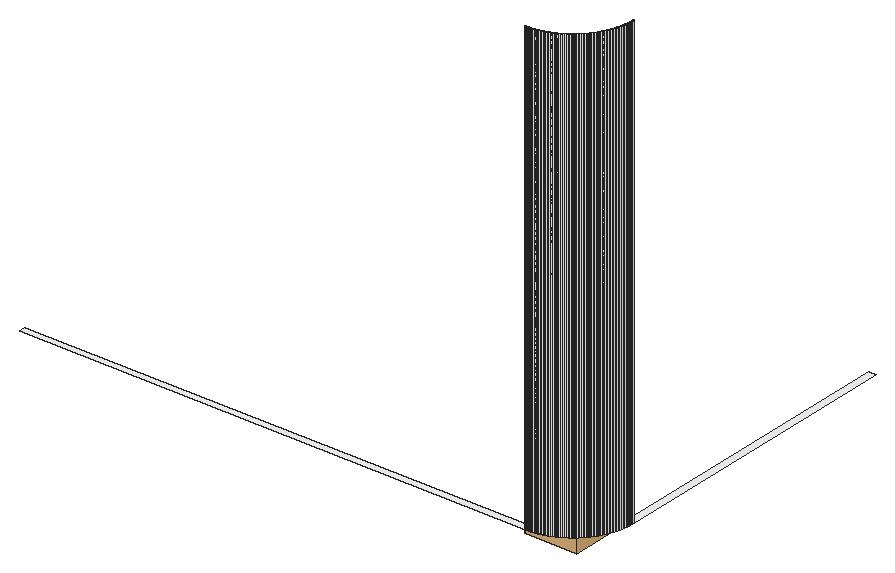
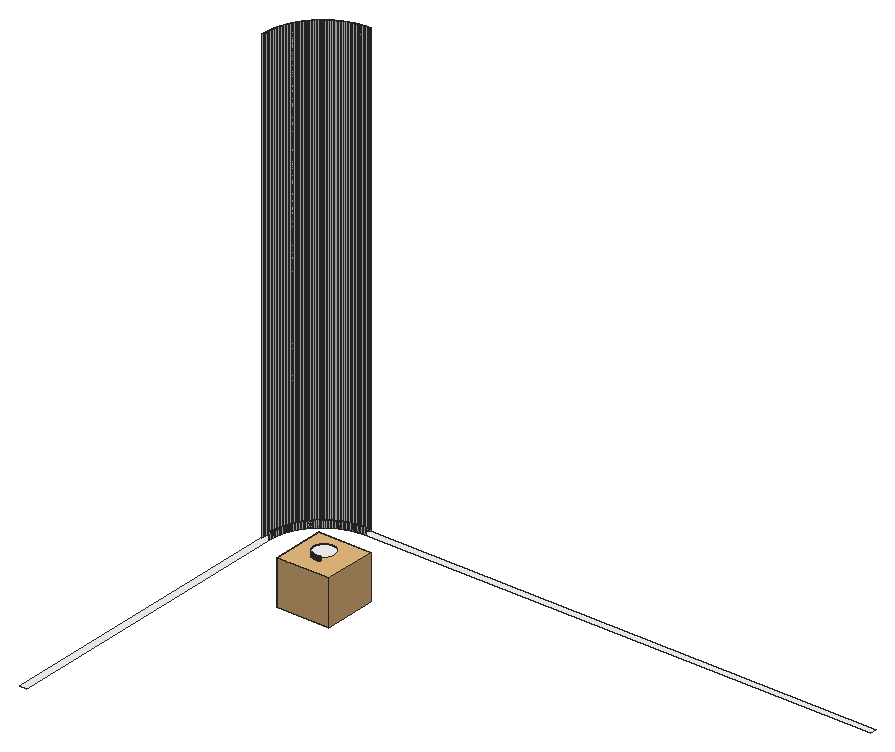
# SketchUp Ruby script. Lengths in inches.
U = 1.inch
M = Sketchup.active_model
def pt(a) = Geom::Point3d.new(a.map { |v| v * U })
def face(e, loops, mat)
  f = e.add_face(loops[0].map { |a| pt(a) })
  loops[1..].each { |l| e.add_face(l.map { |a| pt(a) }).erase! }
  f.material = f.back_material = mat if mat
  f
end
# faces: each face lists its corners as indices into pts; further lists are holes
def faces(e, pts, list, mat = nil) = list.each { |f| face(e, (f[0].is_a?(Array) ? f : [f]).map { |l| l.map { |i| pts[i] } }, mat) }
# xy, xz, yz: faces in a plane at the given z, y or x. An outline is a flat list of corners, or four numbers for a rectangle; further outlines are holes
def ring(l) = l.size == 4 ? [[l[0], l[1]], [l[2], l[1]], [l[2], l[3]], [l[0], l[3]]] : l.each_slice(2).to_a
def flat(e, list, mat, &to3) = list.each { |f| face(e, (f[0].is_a?(Array) ? f : [f]).map { |l| ring(l).map { |u, v| to3.(u, v) } }, mat) }
def xy(e, z, list, mat = nil) = flat(e, list, mat) { |x, y| [x, y, z] }
def xz(e, y, list, mat = nil) = flat(e, list, mat) { |x, z| [x, y, z] }
def yz(e, x, list, mat = nil) = flat(e, list, mat) { |y, z| [x, y, z] }
def lines(e, pts, list) = list.each { |a, b| e.add_line(pt(pts[a]), pt(pts[b])) }
# prism: a flat outline (further loops are holes) pulled along v
def prism(e, loops, v, mat = nil)
  f = face(e, loops, mat); d = Geom::Vector3d.new(v.map { |x| x * U })
  f.pushpull(f.normal.samedirection?(d) ? d.length : -d.length)
end
def box(e, o, s, mat = nil) = prism(e, [[o, [o[0] + s[0], o[1], o[2]], [o[0] + s[0], o[1] + s[1], o[2]], [o[0], o[1] + s[1], o[2]]]], [0, 0, s[2]], mat)
def at(x, y, z, deg = 0) = Geom::Transformation.translation(pt([x, y, z])) * Geom::Transformation.rotation(ORIGIN, Z_AXIS, deg.degrees)
def axes(o, x, y, z) = Geom::Transformation.new([*x, 0, *y, 0, *z, 0, *pt(o).to_a, 1])
def part(name) = M.definitions.add(name)
# library, detail: a bought-in or finely detailed component or shape, given as its bounding box
def library(name, o, s) = part(name).tap { |d| box(d.entities, o, s) }
def detail(e, o, s) = box(e.add_group.entities, o, s)
def put(e, d, t, mat = nil) = e.add_instance(d, t).tap { |i| i.material = mat if mat }
def group(e, t, mat = nil) = e.add_group.tap { |g| g.transformation = t; g.material = mat if mat }.entities
root = M.entities
M.materials.add("[Quartz Light Grey]").color = [251, 251, 252]
c1 = library("5",[-6.25,-6.25,-13.16],[15.58,15.58,13.16])
xy(root,115,[[60,187,60,189,210.21,189,210.42,189.01,210.63,189.01,211.05,189.03,211.26,189.05,211.46,189.07,211.88,189.11,212.3,189.17,212.5,189.2,212.71,189.23,212.92,189.27,213.12,189.31,213.33,189.35,213.53,189.39,213.74,189.44,213.9375,189.49,214.14,189.55,214.34,189.6,214.94,189.78,215.54,189.99,215.73,190.0625,215.93,190.14,216.12,190.22,216.32,190.3,216.51,190.38,217.08,190.65,217.26,190.74,217.45,190.84,217.63,190.9375,217.82,191.04,218,191.14,218.54,191.47,218.71,191.58,218.89,191.7,219.0625,191.8125,219.23,191.93,219.4,192.06,219.57,192.18,219.74,192.31,219.91,192.43,220.07,192.57,220.39,192.83,220.71,193.11,221.01,193.39,221.16,193.54,221.3125,193.6875,221.46,193.84,221.61,193.99,221.89,194.29,222.17,194.61,222.43,194.93,222.57,195.09,222.69,195.26,222.82,195.43,222.94,195.6,223.07,195.77,223.1875,195.9375,223.3,196.11,223.42,196.29,223.53,196.46,223.86,197,223.96,197.18,224.0625,197.37,224.16,197.55,224.26,197.74,224.35,197.92,224.62,198.49,224.7,198.68,224.78,198.88,224.86,199.07,224.9375,199.27,225.01,199.46,225.22,200.06,225.4,200.66,225.45,200.86,225.51,201.0625,225.56,201.26,225.61,201.47,225.65,201.67,225.69,201.88,225.73,202.08,225.77,202.29,225.8,202.5,225.83,202.7,225.89,203.12,225.93,203.54,225.95,203.74,225.97,203.95,225.99,204.37,225.99,204.58,226,204.79,226,295,228,295,228,204.76,227.99,204.53,227.99,204.29,227.98,204.06,227.96,203.82,227.94,203.59,227.92,203.35,227.9,203.12,227.875,202.88,227.85,202.65,227.8125,202.42,227.78,202.18,227.7,201.72,227.65,201.49,227.61,201.26,227.56,201.03,227.5,200.8,227.45,200.57,227.39,200.34,227.32,200.11,227.26,199.89,227.19,199.66,227.12,199.4375,227.04,199.21,226.97,198.99,226.89,198.77,226.8,198.55,226.72,198.33,226.54,197.89,226.44,197.68,226.35,197.46,226.25,197.25,226.14,197.04,226.04,196.83,225.82,196.41,225.7,196.2,225.59,196,225.35,195.6,225.22,195.39,225.1,195.2,224.97,195,224.83,194.8,224.7,194.61,224.5625,194.42,224.42,194.23,224.28,194.04,224.14,193.86,223.99,193.67,223.84,193.49,223.6875,193.31,223.53,193.13,223.375,192.96,223.22,192.78,223.06,192.61,222.89,192.44,222.73,192.27,222.56,192.11,222.39,191.94,222.22,191.78,222.04,191.625,221.87,191.47,221.69,191.3125,221.51,191.16,221.33,191.01,221.14,190.86,220.96,190.72,220.77,190.58,220.58,190.4375,220.39,190.3,220.2,190.17,220,190.03,219.8,189.9,219.61,189.78,219.4,189.65,219,189.41,218.8,189.3,218.59,189.18,218.17,188.96,217.96,188.86,217.75,188.75,217.54,188.65,217.32,188.56,217.11,188.46,216.67,188.28,216.45,188.2,216.23,188.11,216.01,188.03,215.79,187.96,215.5625,187.88,215.34,187.81,215.11,187.74,214.89,187.68,214.66,187.61,214.43,187.55,214.2,187.5,213.97,187.44,213.74,187.39,213.51,187.35,213.28,187.3,212.82,187.22,212.58,187.1875,212.35,187.15,212.12,187.125,211.88,187.1,211.65,187.08,211.41,187.06,211.18,187.04,210.94,187.02,210.71,187.01,210.47,187.01,210.24,187]],"[Quartz Light Grey]")
xy(root,119.5,[[207.84,204,207.76,204.01,207.6875,204.02,207.61,204.03,207.45,204.05,207.375,204.07,207.3,204.08,207.22,204.1,207.15,204.125,207.07,204.15,207,204.17,206.92,204.2,206.71,204.29,206.64,204.33,206.57,204.36,206.43,204.44,206.37,204.48,206.3,204.53,206.24,204.57,206.17,204.62,205.93,204.82,205.88,204.88,205.82,204.93,205.62,205.17,205.57,205.24,205.53,205.3,205.48,205.37,205.44,205.43,205.36,205.57,205.33,205.64,205.29,205.71,205.2,205.92,205.17,206,205.15,206.07,205.125,206.15,205.1,206.22,205.08,206.3,205.07,206.375,205.05,206.45,205.03,206.61,205.02,206.6875,205.01,206.76,205,206.84,205,207.16,205.01,207.24,205.02,207.3125,205.03,207.39,205.05,207.55,205.07,207.625,205.08,207.7,205.1,207.78,205.125,207.85,205.15,207.93,205.17,208,205.2,208.08,205.29,208.29,205.33,208.36,205.36,208.43,205.44,208.57,205.48,208.63,205.53,208.7,205.57,208.76,205.62,208.83,205.82,209.07,205.88,209.12,205.93,209.18,206.17,209.38,206.24,209.43,206.3,209.47,206.37,209.52,206.43,209.56,206.57,209.64,206.64,209.67,206.71,209.71,206.92,209.8,207,209.83,207.07,209.85,207.15,209.875,207.22,209.9,207.3,209.92,207.375,209.93,207.45,209.95,207.61,209.97,207.6875,209.98,207.76,209.99,207.84,210,208.16,210,208.24,209.99,208.3125,209.98,208.39,209.97,208.55,209.95,208.625,209.93,208.7,209.92,208.78,209.9,208.85,209.875,208.93,209.85,209,209.83,209.08,209.8,209.29,209.71,209.36,209.67,209.43,209.64,209.57,209.56,209.63,209.52,209.7,209.47,209.76,209.43,209.83,209.38,210.07,209.18,210.12,209.12,210.18,209.07,210.38,208.83,210.43,208.76,210.47,208.7,210.52,208.63,210.56,208.57,210.64,208.43,210.67,208.36,210.71,208.29,210.8,208.08,210.83,208,210.85,207.93,210.875,207.85,210.9,207.78,210.92,207.7,210.93,207.625,210.95,207.55,210.97,207.39,210.98,207.3125,210.99,207.24,211,207.16,211,206.84,210.99,206.76,210.98,206.6875,210.97,206.61,210.95,206.45,210.93,206.375,210.92,206.3,210.9,206.22,210.875,206.15,210.85,206.07,210.83,206,210.8,205.92,210.71,205.71,210.67,205.64,210.64,205.57,210.56,205.43,210.52,205.37,210.47,205.3,210.43,205.24,210.38,205.17,210.18,204.93,210.12,204.88,210.07,204.82,209.83,204.62,209.76,204.57,209.7,204.53,209.63,204.48,209.57,204.44,209.43,204.36,209.36,204.33,209.29,204.29,209.08,204.2,209,204.17,208.93,204.15,208.85,204.125,208.78,204.1,208.7,204.08,208.625,204.07,208.55,204.05,208.39,204.03,208.3125,204.02,208.24,204.01,208.16,204]],"[Quartz Light Grey]")
xz(root,187,[[210,115,210.24,249]],"[Quartz Light Grey]")
xz(root,187.01,[[210.47,115,210.71,249]],"[Quartz Light Grey]")
xz(root,189,[[210,115,210.21,117]],"[Quartz Light Grey]")
xz(root,189.01,[[210.42,115,210.63,117]],"[Quartz Light Grey]")
xz(root,204,[[207.84,117,207.92,119.5],[207.92,117,208,119.5],[208,117,208.08,119.5],[208.08,117,208.16,119.5]],"[Quartz Light Grey]")
xz(root,210,[[207.84,117,207.92,119.5],[207.92,117,208,119.5],[208,117,208.08,119.5],[208.08,117,208.16,119.5]],"[Quartz Light Grey]")
yz(root,211,[[206.84,117,206.92,119.5],[206.92,117,207,119.5],[207,117,207.08,119.5],[207.08,117,207.16,119.5]],"[Quartz Light Grey]")
yz(root,225.99,[[204.37,115,204.58,117]],"[Quartz Light Grey]")
yz(root,226,[[204.79,115,205,117]],"[Quartz Light Grey]")
yz(root,227.99,[[204.29,115,204.53,249]],"[Quartz Light Grey]")
yz(root,228,[[204.76,115,205,249]],"[Quartz Light Grey]")
p = [[210.24,187,115],[210.47,187.01,115],[210.47,187.01,249],[210.24,187,249],[210.71,187.01,115],[210.94,187.02,115],
  [210.94,187.02,249],[210.71,187.01,249],[211.18,187.04,115],[211.18,187.04,249],[211.41,187.06,115],[211.41,187.06,249],
  [211.65,187.08,115],[211.65,187.08,249],[211.88,187.1,115],[211.88,187.1,249],[212.12,187.125,115],[212.12,187.125,249],
  [212.35,187.15,115],[212.35,187.15,249],[212.58,187.1875,115],[212.58,187.1875,249],[212.82,187.22,115],[212.82,187.22,249],
  [213.05,187.26,115],[213.05,187.26,249],[213.28,187.3,115],[213.28,187.3,249],[213.51,187.35,115],[213.51,187.35,249],
  [213.74,187.39,115],[213.74,187.39,249],[213.97,187.44,115],[213.97,187.44,249],[214.2,187.5,115],[214.2,187.5,249],
  [214.43,187.55,115],[214.43,187.55,249],[214.66,187.61,115],[214.66,187.61,249],[214.89,187.68,115],[214.89,187.68,249],
  [215.11,187.74,115],[215.11,187.74,249],[215.34,187.81,115],[215.34,187.81,249],[215.5625,187.88,115],[215.5625,187.88,249],
  [215.79,187.96,115],[215.79,187.96,249],[216.01,188.03,115],[216.01,188.03,249],[216.23,188.11,115],[216.23,188.11,249],
  [216.45,188.2,115],[216.45,188.2,249],[216.67,188.28,115],[216.67,188.28,249],[216.89,188.37,115],[216.89,188.37,249],
  [217.11,188.46,115],[217.11,188.46,249],[217.32,188.56,115],[217.32,188.56,249],[217.54,188.65,115],[217.54,188.65,249],
  [217.75,188.75,115],[217.75,188.75,249],[217.96,188.86,115],[217.96,188.86,249],[218.17,188.96,115],[218.17,188.96,249],
  [210.42,189.01,115],[210.21,189,115],[210.21,189,117],[210.42,189.01,117],[210.84,189.02,115],[210.63,189.01,115],
  [210.63,189.01,117],[210.84,189.02,117],[211.05,189.03,115],[211.05,189.03,117],[211.26,189.05,115],[211.26,189.05,117],
  [211.46,189.07,115],[211.46,189.07,117],[218.38,189.07,115],[218.38,189.07,249],[211.67,189.09,115],[211.67,189.09,117],
  [211.88,189.11,115],[211.88,189.11,117],[212.09,189.14,115],[212.09,189.14,117],[212.3,189.17,115],[212.3,189.17,117],
  [218.59,189.18,115],[218.59,189.18,249],[212.5,189.2,115],[212.5,189.2,117],[212.71,189.23,115],[212.71,189.23,117],
  [212.92,189.27,115],[212.92,189.27,117],[218.8,189.3,115],[218.8,189.3,249],[213.12,189.31,115],[213.12,189.31,117],
  [213.33,189.35,115],[213.33,189.35,117],[213.53,189.39,115],[213.53,189.39,117],[219,189.41,115],[219,189.41,249],
  [213.74,189.44,115],[213.74,189.44,117],[213.9375,189.49,115],[213.9375,189.49,117],[219.2,189.53,115],[219.2,189.53,249],
  [214.14,189.55,115],[214.14,189.55,117],[214.34,189.6,115],[214.34,189.6,117],[219.4,189.65,115],[219.4,189.65,249],
  [214.54,189.66,115],[214.54,189.66,117],[214.74,189.72,115],[214.74,189.72,117],[214.94,189.78,115],[214.94,189.78,117],
  [219.61,189.78,115],[219.61,189.78,249],[215.14,189.85,115],[215.14,189.85,117],[215.34,189.92,115],[215.34,189.92,117],
  [219.8,189.9,115],[219.8,189.9,249],[215.54,189.99,115],[215.54,189.99,117],[220,190.03,115],[220,190.03,249],
  [215.73,190.0625,115],[215.73,190.0625,117],[220.2,190.17,115],[220.2,190.17,249],[215.93,190.14,115],[215.93,190.14,117],
  [216.12,190.22,115],[216.12,190.22,117],[216.32,190.3,115],[216.32,190.3,117],[220.39,190.3,115],[220.39,190.3,249],
  [216.51,190.38,115],[216.51,190.38,117],[220.58,190.4375,115],[220.58,190.4375,249],[216.7,190.47,115],[216.7,190.47,117],
  [220.77,190.58,115],[220.77,190.58,249],[216.89,190.56,115],[216.89,190.56,117],[217.08,190.65,115],[217.08,190.65,117],
  [220.96,190.72,115],[220.96,190.72,249],[217.26,190.74,115],[217.26,190.74,117],[217.45,190.84,115],[217.45,190.84,117],
  [221.14,190.86,115],[221.14,190.86,249],[217.63,190.9375,115],[217.63,190.9375,117],[217.82,191.04,115],[217.82,191.04,117],
  [221.33,191.01,115],[221.33,191.01,249],[218,191.14,115],[218,191.14,117],[221.51,191.16,115],[221.51,191.16,249],
  [218.18,191.25,115],[218.18,191.25,117],[218.36,191.36,115],[218.36,191.36,117],[221.69,191.3125,115],[221.69,191.3125,249],
  [221.87,191.47,115],[221.87,191.47,249],[218.54,191.47,115],[218.54,191.47,117],[218.71,191.58,115],[218.71,191.58,117],
  [222.04,191.625,115],[222.04,191.625,249],[218.89,191.7,115],[218.89,191.7,117],[222.22,191.78,115],[222.22,191.78,249],
  [219.0625,191.8125,115],[219.0625,191.8125,117],[219.23,191.93,115],[219.23,191.93,117],[222.39,191.94,115],[222.39,191.94,249],
  [219.4,192.06,115],[219.4,192.06,117],[222.56,192.11,115],[222.56,192.11,249],[219.57,192.18,115],[219.57,192.18,117],
  [222.73,192.27,115],[222.73,192.27,249],[219.74,192.31,115],[219.74,192.31,117],[219.91,192.43,115],[219.91,192.43,117],
  [222.89,192.44,115],[222.89,192.44,249],[220.07,192.57,115],[220.07,192.57,117],[223.06,192.61,115],[223.06,192.61,249],
  [220.23,192.7,115],[220.23,192.7,117],[223.22,192.78,115],[223.22,192.78,249],[220.39,192.83,115],[220.39,192.83,117],
  [220.55,192.97,115],[220.55,192.97,117],[223.375,192.96,115],[223.375,192.96,249],[220.71,193.11,115],[220.71,193.11,117],
  [223.53,193.13,115],[223.53,193.13,249],[220.86,193.25,115],[220.86,193.25,117],[223.6875,193.31,115],[223.6875,193.31,249],
  [221.01,193.39,115],[221.01,193.39,117],[223.84,193.49,115],[223.84,193.49,249],[221.16,193.54,115],[221.16,193.54,117],
  [221.3125,193.6875,115],[221.3125,193.6875,117],[223.99,193.67,115],[223.99,193.67,249],[221.46,193.84,115],[221.46,193.84,117],
  [224.14,193.86,115],[224.14,193.86,249],[221.61,193.99,115],[221.61,193.99,117],[224.28,194.04,115],[224.28,194.04,249],
  [221.75,194.14,115],[221.75,194.14,117],[224.42,194.23,115],[224.42,194.23,249],[221.89,194.29,115],[221.89,194.29,117],
  [224.5625,194.42,115],[224.5625,194.42,249],[222.03,194.45,115],[222.03,194.45,117],[224.7,194.61,115],[224.7,194.61,249],
  [222.17,194.61,115],[222.17,194.61,117],[222.3,194.77,115],[222.3,194.77,117],[224.83,194.8,115],[224.83,194.8,249],
  [222.43,194.93,115],[222.43,194.93,117],[224.97,195,115],[224.97,195,249],[222.57,195.09,115],[222.57,195.09,117],
  [225.1,195.2,115],[225.1,195.2,249],[222.69,195.26,115],[222.69,195.26,117],[225.22,195.39,115],[225.22,195.39,249],
  [222.82,195.43,115],[222.82,195.43,117],[222.94,195.6,115],[222.94,195.6,117],[225.35,195.6,115],[225.35,195.6,249],
  [223.07,195.77,115],[223.07,195.77,117],[225.47,195.8,115],[225.47,195.8,249],[223.1875,195.9375,115],[223.1875,195.9375,117],
  [225.59,196,115],[225.59,196,249],[223.3,196.11,115],[223.3,196.11,117],[225.7,196.2,115],[225.7,196.2,249],
  [223.42,196.29,115],[223.42,196.29,117],[225.82,196.41,115],[225.82,196.41,249],[223.53,196.46,115],[223.53,196.46,117],
  [225.93,196.62,115],[225.93,196.62,249],[223.64,196.64,115],[223.64,196.64,117],[223.75,196.82,115],[223.75,196.82,117],
  [226.04,196.83,115],[226.04,196.83,249],[223.86,197,115],[223.86,197,117],[226.14,197.04,115],[226.14,197.04,249],
  [223.96,197.18,115],[223.96,197.18,117],[226.25,197.25,115],[226.25,197.25,249],[224.0625,197.37,115],[224.0625,197.37,117],
  [226.35,197.46,115],[226.35,197.46,249],[224.16,197.55,115],[224.16,197.55,117],[226.44,197.68,115],[226.44,197.68,249],
  [224.26,197.74,115],[224.26,197.74,117],[224.35,197.92,115],[224.35,197.92,117],[226.54,197.89,115],[226.54,197.89,249],
  [224.44,198.11,115],[224.44,198.11,117],[226.63,198.11,115],[226.63,198.11,249],[224.53,198.3,115],[224.53,198.3,117],
  [226.72,198.33,115],[226.72,198.33,249],[224.62,198.49,115],[224.62,198.49,117],[226.8,198.55,115],[226.8,198.55,249],
  [224.7,198.68,115],[224.7,198.68,117],[226.89,198.77,115],[226.89,198.77,249],[224.78,198.88,115],[224.78,198.88,117],
  [226.97,198.99,115],[226.97,198.99,249],[224.86,199.07,115],[224.86,199.07,117],[227.04,199.21,115],[227.04,199.21,249],
  [224.9375,199.27,115],[224.9375,199.27,117],[227.12,199.4375,115],[227.12,199.4375,249],[225.01,199.46,115],[225.01,199.46,117],
  [227.19,199.66,115],[227.19,199.66,249],[225.08,199.66,115],[225.08,199.66,117],[225.15,199.86,115],[225.15,199.86,117],
  [227.26,199.89,115],[227.26,199.89,249],[225.22,200.06,115],[225.22,200.06,117],[227.32,200.11,115],[227.32,200.11,249],
  [225.28,200.26,115],[225.28,200.26,117],[227.39,200.34,115],[227.39,200.34,249],[225.34,200.46,115],[225.34,200.46,117],
  [227.45,200.57,115],[227.45,200.57,249],[225.4,200.66,115],[225.4,200.66,117],[227.5,200.8,115],[227.5,200.8,249],
  [225.45,200.86,115],[225.45,200.86,117],[227.56,201.03,115],[227.56,201.03,249],[225.51,201.0625,115],[225.51,201.0625,117],
  [227.61,201.26,115],[227.61,201.26,249],[225.56,201.26,115],[225.56,201.26,117],[225.61,201.47,115],[225.61,201.47,117],
  [227.65,201.49,115],[227.65,201.49,249],[225.65,201.67,115],[225.65,201.67,117],[227.7,201.72,115],[227.7,201.72,249],
  [225.69,201.88,115],[225.69,201.88,117],[227.74,201.95,115],[227.74,201.95,249],[225.73,202.08,115],[225.73,202.08,117],
  [227.78,202.18,115],[227.78,202.18,249],[225.77,202.29,115],[225.77,202.29,117],[227.8125,202.42,115],[227.8125,202.42,249],
  [225.8,202.5,115],[225.8,202.5,117],[227.85,202.65,115],[227.85,202.65,249],[225.83,202.7,115],[225.83,202.7,117],
  [225.86,202.91,115],[225.86,202.91,117],[227.875,202.88,115],[227.875,202.88,249],[225.89,203.12,115],[225.89,203.12,117],
  [227.9,203.12,115],[227.9,203.12,249],[225.91,203.33,115],[225.91,203.33,117],[227.92,203.35,115],[227.92,203.35,249],
  [225.93,203.54,115],[225.93,203.54,117],[227.94,203.59,115],[227.94,203.59,249],[225.95,203.74,115],[225.95,203.74,117],
  [227.96,203.82,115],[227.96,203.82,249],[225.97,203.95,115],[225.97,203.95,117],[227.98,204.06,115],[227.98,204.06,249],
  [225.98,204.16,115],[225.98,204.16,117],[227.99,204.29,115],[227.99,204.29,249],[225.99,204.37,115],[225.99,204.37,117],
  [227.99,204.53,115],[228,204.76,115],[228,204.76,249],[227.99,204.53,249],[226,204.79,115],[225.99,204.58,115],
  [225.99,204.58,117],[226,204.79,117],[207.53,204.04,117],[207.45,204.05,117],[207.45,204.05,119.5],[207.53,204.04,119.5],
  [207.61,204.03,117],[207.61,204.03,119.5],[207.6875,204.02,117],[207.6875,204.02,119.5],[207.76,204.01,117],[207.76,204.01,119.5],
  [207.84,204,117],[207.84,204,119.5],[208.24,204.01,117],[208.16,204,117],[208.16,204,119.5],[208.24,204.01,119.5],
  [208.3125,204.02,117],[208.3125,204.02,119.5],[208.39,204.03,117],[208.39,204.03,119.5],[208.47,204.04,117],[208.47,204.04,119.5],
  [208.55,204.05,117],[208.55,204.05,119.5],[207.07,204.15,117],[207,204.17,117],[207,204.17,119.5],[207.07,204.15,119.5],
  [207.15,204.125,117],[207.15,204.125,119.5],[207.22,204.1,117],[207.22,204.1,119.5],[207.3,204.08,117],[207.3,204.08,119.5],
  [207.375,204.07,117],[207.375,204.07,119.5],[208.625,204.07,117],[208.625,204.07,119.5],[208.7,204.08,117],[208.7,204.08,119.5],
  [208.78,204.1,117],[208.78,204.1,119.5],[208.85,204.125,117],[208.85,204.125,119.5],[208.93,204.15,117],[208.93,204.15,119.5],
  [209,204.17,117],[209,204.17,119.5],[206.85,204.23,117],[206.78,204.26,117],[206.78,204.26,119.5],[206.85,204.23,119.5],
  [206.92,204.2,117],[206.92,204.2,119.5],[209.08,204.2,117],[209.08,204.2,119.5],[209.15,204.23,117],[209.15,204.23,119.5],
  [209.22,204.26,117],[209.22,204.26,119.5],[206.71,204.29,117],[206.64,204.33,117],[206.64,204.33,119.5],[206.71,204.29,119.5],
  [209.29,204.29,117],[209.29,204.29,119.5],[209.36,204.33,117],[209.36,204.33,119.5],[209.43,204.36,117],[209.43,204.36,119.5],
  [209.5,204.4,117],[209.5,204.4,119.5],[209.57,204.44,117],[209.57,204.44,119.5],[209.63,204.48,117],[209.63,204.48,119.5],
  [209.7,204.53,117],[209.7,204.53,119.5],[209.76,204.57,117],[209.76,204.57,119.5],[209.83,204.62,117],[209.83,204.62,119.5],
  [209.89,204.67,117],[209.89,204.67,119.5],[209.95,204.72,117],[209.95,204.72,119.5],[210.01,204.77,117],[210.01,204.77,119.5],
  [210.07,204.82,117],[210.07,204.82,119.5],[210.12,204.88,117],[210.12,204.88,119.5],[210.18,204.93,117],[210.18,204.93,119.5],
  [210.23,204.99,117],[210.23,204.99,119.5],[210.28,205.05,117],[210.28,205.05,119.5],[210.33,205.11,117],[210.33,205.11,119.5],
  [210.38,205.17,117],[210.38,205.17,119.5],[210.43,205.24,117],[210.43,205.24,119.5],[210.47,205.3,117],[210.47,205.3,119.5],
  [210.52,205.37,117],[210.52,205.37,119.5],[210.56,205.43,117],[210.56,205.43,119.5],[210.6,205.5,117],[210.6,205.5,119.5],
  [210.64,205.57,117],[210.64,205.57,119.5],[210.67,205.64,117],[210.67,205.64,119.5],[210.71,205.71,117],[210.71,205.71,119.5],
  [210.74,205.78,117],[210.74,205.78,119.5],[210.77,205.85,117],[210.77,205.85,119.5],[210.8,205.92,117],[210.8,205.92,119.5],
  [210.83,206,117],[210.83,206,119.5],[210.85,206.07,117],[210.85,206.07,119.5],[210.875,206.15,117],[210.875,206.15,119.5],
  [210.9,206.22,117],[210.9,206.22,119.5],[210.92,206.3,117],[210.92,206.3,119.5],[210.93,206.375,117],[210.93,206.375,119.5],
  [210.95,206.45,117],[210.95,206.45,119.5],[210.96,206.53,117],[210.96,206.53,119.5],[210.97,206.61,117],[210.97,206.61,119.5],
  [210.98,206.6875,117],[210.98,206.6875,119.5],[210.99,206.76,117],[210.99,206.76,119.5],[211,206.84,117],[211,206.84,119.5],
  [210.98,207.3125,117],[210.99,207.24,117],[210.99,207.24,119.5],[210.98,207.3125,119.5],[211,207.16,117],[211,207.16,119.5],
  [210.97,207.39,117],[210.97,207.39,119.5],[210.96,207.47,117],[210.96,207.47,119.5],[210.93,207.625,117],[210.95,207.55,117],
  [210.95,207.55,119.5],[210.93,207.625,119.5],[210.92,207.7,117],[210.92,207.7,119.5],[210.9,207.78,117],[210.9,207.78,119.5],
  [210.875,207.85,117],[210.875,207.85,119.5],[210.83,208,117],[210.85,207.93,117],[210.85,207.93,119.5],[210.83,208,119.5],
  [210.8,208.08,117],[210.8,208.08,119.5],[210.74,208.22,117],[210.77,208.15,117],[210.77,208.15,119.5],[210.74,208.22,119.5],
  [210.71,208.29,117],[210.71,208.29,119.5],[210.67,208.36,117],[210.67,208.36,119.5],[210.6,208.5,117],[210.64,208.43,117],
  [210.64,208.43,119.5],[210.6,208.5,119.5],[210.56,208.57,117],[210.56,208.57,119.5],[210.47,208.7,117],[210.52,208.63,117],
  [210.52,208.63,119.5],[210.47,208.7,119.5],[210.43,208.76,117],[210.43,208.76,119.5],[210.33,208.89,117],[210.38,208.83,117],
  [210.38,208.83,119.5],[210.33,208.89,119.5],[210.23,209.01,117],[210.28,208.95,117],[210.28,208.95,119.5],[210.23,209.01,119.5],
  [210.18,209.07,117],[210.18,209.07,119.5],[210.07,209.18,117],[210.12,209.12,117],[210.12,209.12,119.5],[210.07,209.18,119.5],
  [209.95,209.28,117],[210.01,209.23,117],[210.01,209.23,119.5],[209.95,209.28,119.5],[209.83,209.38,117],[209.89,209.33,117],
  [209.89,209.33,119.5],[209.83,209.38,119.5],[209.7,209.47,117],[209.76,209.43,117],[209.76,209.43,119.5],[209.7,209.47,119.5],
  [209.57,209.56,117],[209.63,209.52,117],[209.63,209.52,119.5],[209.57,209.56,119.5],[209.36,209.67,117],[209.43,209.64,117],
  [209.43,209.64,119.5],[209.36,209.67,119.5],[209.5,209.6,117],[209.5,209.6,119.5],[206.71,209.71,117],[206.78,209.74,117],
  [206.78,209.74,119.5],[206.71,209.71,119.5],[206.85,209.77,117],[206.85,209.77,119.5],[209.15,209.77,117],[209.22,209.74,117],
  [209.22,209.74,119.5],[209.15,209.77,119.5],[209.29,209.71,117],[209.29,209.71,119.5],[206.92,209.8,117],[206.92,209.8,119.5],
  [207,209.83,117],[207,209.83,119.5],[207.07,209.85,117],[207.07,209.85,119.5],[208.93,209.85,117],[209,209.83,117],
  [209,209.83,119.5],[208.93,209.85,119.5],[209.08,209.8,117],[209.08,209.8,119.5],[207.15,209.875,117],[207.15,209.875,119.5],
  [207.22,209.9,117],[207.22,209.9,119.5],[207.3,209.92,117],[207.3,209.92,119.5],[207.375,209.93,117],[207.375,209.93,119.5],
  [207.45,209.95,117],[207.45,209.95,119.5],[207.53,209.96,117],[207.53,209.96,119.5],[208.47,209.96,117],[208.55,209.95,117],
  [208.55,209.95,119.5],[208.47,209.96,119.5],[208.625,209.93,117],[208.625,209.93,119.5],[208.7,209.92,117],[208.7,209.92,119.5],
  [208.78,209.9,117],[208.78,209.9,119.5],[208.85,209.875,117],[208.85,209.875,119.5],[207.61,209.97,117],[207.61,209.97,119.5],
  [207.6875,209.98,117],[207.6875,209.98,119.5],[207.76,209.99,117],[207.76,209.99,119.5],[207.84,210,117],[207.84,210,119.5],
  [208.16,210,117],[208.24,209.99,117],[208.24,209.99,119.5],[208.16,210,119.5],[208.3125,209.98,117],[208.3125,209.98,119.5],
  [208.39,209.97,117],[208.39,209.97,119.5],[210,187,117],[210,189,117]]
faces(root,p,[[0,1,2,3],[4,5,6,7],[5,8,9,6],[8,10,11,9],[10,12,13,11],[12,14,15,13],[14,16,17,15],[16,18,19,17],
  [18,20,21,19],[20,22,23,21],[22,24,25,23],[24,26,27,25],[26,28,29,27],[28,30,31,29],[30,32,33,31],[32,34,35,33],
  [34,36,37,35],[36,38,39,37],[38,40,41,39],[40,42,43,41],[42,44,45,43],[44,46,47,45],[46,48,49,47],[48,50,51,49],
  [50,52,53,51],[52,54,55,53],[54,56,57,55],[56,58,59,57],[58,60,61,59],[60,62,63,61],[62,64,65,63],[64,66,67,65],
  [66,68,69,67],[68,70,71,69],[72,73,74,75],[76,77,78,79],[80,76,79,81],[82,80,81,83],[84,82,83,85],[70,86,87,71],
  [88,84,85,89],[90,88,89,91],[92,90,91,93],[94,92,93,95],[86,96,97,87],[98,94,95,99],[100,98,99,101],[102,100,101,103],
  [96,104,105,97],[106,102,103,107],[108,106,107,109],[110,108,109,111],[104,112,113,105],[114,110,111,115],[116,114,115,117],[112,118,119,113],
  [120,116,117,121],[122,120,121,123],[118,124,125,119],[126,122,123,127],[128,126,127,129],[130,128,129,131],[124,132,133,125],[134,130,131,135],
  [136,134,135,137],[132,138,139,133],[140,136,137,141],[138,142,143,139],[144,140,141,145],[142,146,147,143],[148,144,145,149],[150,148,149,151],
  [152,150,151,153],[146,154,155,147],[156,152,153,157],[154,158,159,155],[160,156,157,161],[158,162,163,159],[164,160,161,165],[166,164,165,167],
  [162,168,169,163],[170,166,167,171],[172,170,171,173],[168,174,175,169],[176,172,173,177],[178,176,177,179],[174,180,181,175],[182,178,179,183],
  [180,184,185,181],[186,182,183,187],[188,186,187,189],[184,190,191,185],[190,192,193,191],[194,188,189,195],[196,194,195,197],[192,198,199,193],
  [200,196,197,201],[198,202,203,199],[204,200,201,205],[206,204,205,207],[202,208,209,203],[210,206,207,211],[208,212,213,209],[214,210,211,215],
  [212,216,217,213],[218,214,215,219],[220,218,219,221],[216,222,223,217],[224,220,221,225],[222,226,227,223],[228,224,225,229],[226,230,231,227],
  [232,228,229,233],[234,232,233,235],[230,236,237,231],[238,234,235,239],[236,240,241,237],[242,238,239,243],[240,244,245,241],[246,242,243,247],
  [244,248,249,245],[250,246,247,251],[252,250,251,253],[248,254,255,249],[256,252,253,257],[254,258,259,255],[260,256,257,261],[258,262,263,259],
  [264,260,261,265],[262,266,267,263],[268,264,265,269],[266,270,271,267],[272,268,269,273],[270,274,275,271],[276,272,273,277],[278,276,277,279],
  [274,280,281,275],[282,278,279,283],[280,284,285,281],[286,282,283,287],[284,288,289,285],[290,286,287,291],[288,292,293,289],[294,290,291,295],
  [296,294,295,297],[292,298,299,293],[300,296,297,301],[298,302,303,299],[304,300,301,305],[302,306,307,303],[308,304,305,309],[306,310,311,307],
  [312,308,309,313],[310,314,315,311],[316,312,313,317],[314,318,319,315],[320,316,317,321],[322,320,321,323],[318,324,325,319],[326,322,323,327],
  [324,328,329,325],[330,326,327,331],[328,332,333,329],[334,330,331,335],[332,336,337,333],[338,334,335,339],[336,340,341,337],[342,338,339,343],
  [344,342,343,345],[340,346,347,341],[348,344,345,349],[346,350,351,347],[352,348,349,353],[350,354,355,351],[356,352,353,357],[354,358,359,355],
  [360,356,357,361],[358,362,363,359],[364,360,361,365],[362,366,367,363],[368,364,365,369],[366,370,371,367],[372,368,369,373],[370,374,375,371],
  [376,372,373,377],[374,378,379,375],[380,376,377,381],[382,380,381,383],[378,384,385,379],[386,382,383,387],[384,388,389,385],[390,386,387,391],
  [388,392,393,389],[394,390,391,395],[392,396,397,393],[398,394,395,399],[396,400,401,397],[402,398,399,403],[400,404,405,401],[406,402,403,407],
  [404,408,409,405],[410,406,407,411],[412,410,411,413],[408,414,415,409],[416,412,413,417],[414,418,419,415],[420,416,417,421],[418,422,423,419],
  [424,420,421,425],[422,426,427,423],[428,424,425,429],[426,430,431,427],[432,428,429,433],[430,434,435,431],[436,432,433,437],[438,436,437,439],
  [434,440,441,435],[442,438,439,443],[440,444,445,441],[446,442,443,447],[444,448,449,445],[450,446,447,451],[448,452,453,449],[454,450,451,455],
  [452,456,457,453],[458,454,455,459],[456,460,461,457],[462,458,459,463],[460,464,465,461],[466,462,463,467],[468,469,470,471],[472,473,474,475],
  [476,477,478,479],[480,476,479,481],[482,480,481,483],[484,482,483,485],[486,484,485,487],[488,489,490,491],[492,488,491,493],[494,492,493,495],
  [496,494,495,497],[498,496,497,499],[500,501,502,503],[504,500,503,505],[506,504,505,507],[508,506,507,509],[510,508,509,511],[477,510,511,478],
  [512,498,499,513],[514,512,513,515],[516,514,515,517],[518,516,517,519],[520,518,519,521],[522,520,521,523],[524,525,526,527],[528,524,527,529],
  [501,528,529,502],[530,522,523,531],[532,530,531,533],[534,532,533,535],[536,537,538,539],[525,536,539,526],[540,534,535,541],[542,540,541,543],
  [544,542,543,545],[546,544,545,547],[548,546,547,549],[550,548,549,551],[552,550,551,553],[554,552,553,555],[556,554,555,557],[558,556,557,559],
  [560,558,559,561],[562,560,561,563],[564,562,563,565],[566,564,565,567],[568,566,567,569],[570,568,569,571],[572,570,571,573],[574,572,573,575],
  [576,574,575,577],[578,576,577,579],[580,578,579,581],[582,580,581,583],[584,582,583,585],[586,584,585,587],[588,586,587,589],[590,588,589,591],
  [592,590,591,593],[594,592,593,595],[596,594,595,597],[598,596,597,599],[600,598,599,601],[602,600,601,603],[604,602,603,605],[606,604,605,607],
  [608,606,607,609],[610,608,609,611],[612,610,611,613],[614,612,613,615],[616,614,615,617],[618,616,617,619],[620,618,619,621],[622,620,621,623],
  [624,625,626,627],[625,628,629,626],[630,624,627,631],[632,630,631,633],[634,635,636,637],[635,632,633,636],[638,634,637,639],[640,638,639,641],
  [642,640,641,643],[644,645,646,647],[645,642,643,646],[648,644,647,649],[650,651,652,653],[651,648,649,652],[654,650,653,655],[656,654,655,657],
  [658,659,660,661],[659,656,657,660],[662,658,661,663],[664,665,666,667],[665,662,663,666],[668,664,667,669],[670,671,672,673],[671,668,669,672],
  [674,675,676,677],[675,670,673,676],[678,674,677,679],[680,681,682,683],[681,678,679,682],[684,685,686,687],[685,680,683,686],[688,689,690,691],
  [689,684,687,690],[692,693,694,695],[693,688,691,694],[696,697,698,699],[697,692,695,698],[700,701,702,703],[701,704,705,702],[704,696,699,705],
  [706,707,708,709],[707,710,711,708],[712,713,714,715],[713,716,717,714],[716,700,703,717],[710,718,719,711],[718,720,721,719],[720,722,723,721],
  [724,725,726,727],[725,728,729,726],[728,712,715,729],[722,730,731,723],[730,732,733,731],[732,734,735,733],[734,736,737,735],[736,738,739,737],
  [738,740,741,739],[742,743,744,745],[743,746,747,744],[746,748,749,747],[748,750,751,749],[750,752,753,751],[752,724,727,753],[740,754,755,741],
  [754,756,757,755],[756,758,759,757],[758,760,761,759],[762,763,764,765],[763,766,767,764],[766,768,769,767],[768,742,745,769]],"[Quartz Light Grey]")
lines(root,p,[[770,771]])
put(root,c1,at(206.46,205.47,118.25),"[Quartz Light Grey]")
